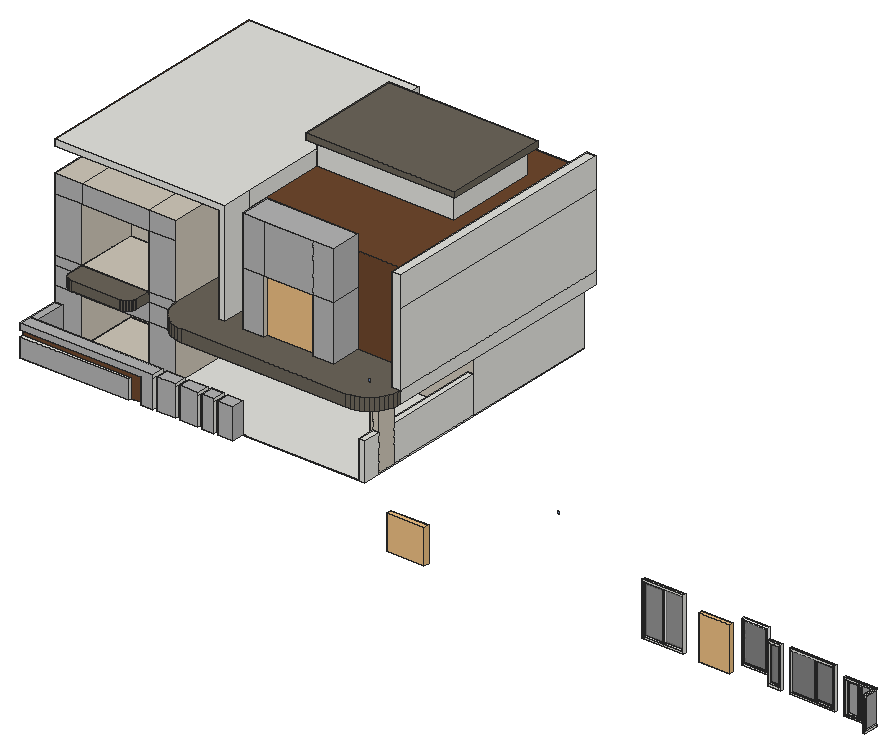
# SketchUp Ruby script. Lengths in millimetres.
U = 1.mm
M = Sketchup.active_model
def pt(a) = Geom::Point3d.new(a.map { |v| v * U })
def face(e, loops, mat)
  f = e.add_face(loops[0].map { |a| pt(a) })
  loops[1..].each { |l| e.add_face(l.map { |a| pt(a) }).erase! }
  f.material = f.back_material = mat if mat
  f
end
# faces: each face lists its corners as indices into pts; further lists are holes
def faces(e, pts, list, mat = nil) = list.each { |f| face(e, (f[0].is_a?(Array) ? f : [f]).map { |l| l.map { |i| pts[i] } }, mat) }
# xy, xz, yz: faces in a plane at the given z, y or x. An outline is a flat list of corners, or four numbers for a rectangle; further outlines are holes
def ring(l) = l.size == 4 ? [[l[0], l[1]], [l[2], l[1]], [l[2], l[3]], [l[0], l[3]]] : l.each_slice(2).to_a
def flat(e, list, mat, &to3) = list.each { |f| face(e, (f[0].is_a?(Array) ? f : [f]).map { |l| ring(l).map { |u, v| to3.(u, v) } }, mat) }
def xy(e, z, list, mat = nil) = flat(e, list, mat) { |x, y| [x, y, z] }
def xz(e, y, list, mat = nil) = flat(e, list, mat) { |x, z| [x, y, z] }
def yz(e, x, list, mat = nil) = flat(e, list, mat) { |y, z| [x, y, z] }
def lines(e, pts, list) = list.each { |a, b| e.add_line(pt(pts[a]), pt(pts[b])) }
# prism: a flat outline (further loops are holes) pulled along v
def prism(e, loops, v, mat = nil)
  f = face(e, loops, mat); d = Geom::Vector3d.new(v.map { |x| x * U })
  f.pushpull(f.normal.samedirection?(d) ? d.length : -d.length)
end
def box(e, o, s, mat = nil) = prism(e, [[o, [o[0] + s[0], o[1], o[2]], [o[0] + s[0], o[1] + s[1], o[2]], [o[0], o[1] + s[1], o[2]]]], [0, 0, s[2]], mat)
def at(x, y, z, deg = 0) = Geom::Transformation.translation(pt([x, y, z])) * Geom::Transformation.rotation(ORIGIN, Z_AXIS, deg.degrees)
def axes(o, x, y, z) = Geom::Transformation.new([*x, 0, *y, 0, *z, 0, *pt(o).to_a, 1])
def part(name) = M.definitions.add(name)
# library, detail: a bought-in or finely detailed component or shape, given as its bounding box
def library(name, o, s) = part(name).tap { |d| box(d.entities, o, s) }
def detail(e, o, s) = box(e.add_group.entities, o, s)
def put(e, d, t, mat = nil) = e.add_instance(d, t).tap { |i| i.material = mat if mat }
def group(e, t, mat = nil) = e.add_group.tap { |g| g.transformation = t; g.material = mat if mat }.entities
root = M.entities
M.materials.add("[0134_DimGray]").color = [107, 101, 90]
M.materials.add("[Beadboard]").color = [109, 71, 45]
M.materials.add("[Carrera Marble]").color = [180, 180, 180]
M.materials.add("[Cinder Block]").color = [206, 198, 184]
M.materials.add("[Color M00]").color = [255, 255, 255]
M.materials.add("[Translucent Glass Gray]1").color = [128, 128, 128]
M.materials["[Translucent Glass Gray]1"].alpha = 0.9
M.materials.add("[Translucent Resin Crush Gray]").color = [165, 165, 165]
M.materials["[Translucent Resin Crush Gray]"].alpha = 1
M.materials.add("[Translucent_Glass_Blue]").color = [100, 149, 237]
M.materials["[Translucent_Glass_Blue]"].alpha = 0.5
c1 = part("Casement window")
xy(c1.entities,0,[[0,0,0,1540,740,1540,740,1440,100,1440,100,0]])
xy(c1.entities,45,[[30,80,100,80,100,1440,660,1440,660,1510,30,1510,30,790,80,790,80,745,30,745]])
xy(c1.entities,70,[[25,815,30,815,30,1510,635,1510,635,1515,25,1515]])
xy(c1.entities,80,[[0,80,10,745],[0,790,10,1540]])
xy(c1.entities,105,[[10,815,15,815,15,1525,635,1525,635,1540,10,1540]])
xy(c1.entities,130,[[25,165,30,660]])
xy(c1.entities,140,[[10,140,15,685]])
xy(c1.entities,1550,[[25,165,30,660]])
xy(c1.entities,1575,[[10,140,15,685]])
xy(c1.entities,1610,[[10,815,10,1540,635,1540,635,1525,15,1525,15,815],[25,815,25,1515,635,1515,635,1510,30,1510,30,815]])
xy(c1.entities,1635,[[0,80,10,745],[30,80,30,745,80,745,80,790,30,790,30,1510,660,1510,660,1440,100,1440,100,80],[0,790,10,1540]])
xy(c1.entities,1715,[[0,0,100,0,100,1440,740,1440,740,1540,0,1540]])
xz(c1.entities,0,[[0,0,100,1715]])
xz(c1.entities,80,[[30,45,100,1635],[0,80,10,1635]])
xz(c1.entities,140,[[10,140,15,1575]])
xz(c1.entities,165,[[25,130,30,1550]])
xz(c1.entities,660,[[25,130,30,1550]])
xz(c1.entities,685,[[10,140,15,1575]])
xz(c1.entities,745,[[30,45,80,1635],[0,80,10,1635]])
xz(c1.entities,790,[[30,45,80,1635],[0,80,10,1635]])
xz(c1.entities,815,[[25,70,30,1610],[10,105,15,1610]])
xz(c1.entities,1440,[[100,0,740,0,740,1715,100,1715,100,1635,660,1635,660,45,100,45]])
xz(c1.entities,1510,[[30,45,660,45,660,1635,30,1635,30,1610,635,1610,635,70,30,70]])
xz(c1.entities,1515,[[25,70,635,1610]],"[Translucent Resin Crush Gray]")
xz(c1.entities,1525,[[15,105,635,1610]],"[Translucent Resin Crush Gray]")
xz(c1.entities,1540,[[0,0,0,80,660,80,660,1635,0,1635,0,1715,740,1715,740,0],[10,80,10,105,635,105,635,1610,10,1610,10,1635,660,1635,660,80]])
yz(c1.entities,0,[[0,0,0,1715,1540,1715,1540,1635,80,1635,80,80,1540,80,1540,0],[745,80,790,1635]])
yz(c1.entities,10,[[[80,80,745,1635],[105,105,720,1610]],[790,80,790,1635,1540,1635,1540,1610,815,1610,815,105,1540,105,1540,80],[[105,105,720,1610],[140,140,685,1575]]])
yz(c1.entities,15,[[815,105,1525,1610],[140,140,685,1575]],"[Translucent Resin Crush Gray]")
yz(c1.entities,25,[[815,70,1515,1610],[165,130,660,1550]],"[Translucent Resin Crush Gray]")
yz(c1.entities,30,[[[80,45,745,1635],[105,70,720,1610]],[790,45,1510,45,1510,70,815,70,815,1610,1510,1610,1510,1635,790,1635],[[105,70,720,1610],[165,130,660,1550]]])
yz(c1.entities,80,[[745,45,790,1635]])
yz(c1.entities,100,[[0,0,1440,0,1440,45,80,45,80,1635,1440,1635,1440,1715,0,1715]])
yz(c1.entities,635,[[1510,70,1515,1610],[1525,105,1540,1610]])
yz(c1.entities,660,[[1440,45,1510,1635]])
yz(c1.entities,740,[[1440,0,1540,1715]])
c2 = library("Group\#97",[0,0,0],[170,1568,2200])
c3 = part("Glass Window Glass Door white frame ประตู หน้าต่าง กรอบขาว")
put(c3.entities,c1,at(10682.2,-611.8,600,-90))
put(c3.entities,c2,at(2888.8,110,0,-90))
g1 = group(c3.entities,at(6847.1,-591.8,600,-90))
xy(g1,0,[[0,0,120,670]])
xy(g1,80,[[0,80,20,590],[50,80,120,590]])
xy(g1,105,[[20,105,25,565],[45,105,50,565]])
xy(g1,170,[[25,170,30,500],[40,170,45,500]])
xy(g1,1860,[[25,170,30,500],[40,170,45,500]])
xy(g1,1925,[[20,105,25,565],[45,105,50,565]])
xy(g1,1950,[[0,80,20,590],[50,80,120,590]])
xy(g1,2030,[[0,0,120,670]])
xz(g1,0,[[0,0,120,2030]])
xz(g1,80,[[0,80,20,1950],[50,80,120,1950]])
xz(g1,105,[[20,105,25,1925],[45,105,50,1925]])
xz(g1,170,[[25,170,30,1860],[40,170,45,1860]])
xz(g1,500,[[25,170,30,1860],[40,170,45,1860]])
xz(g1,565,[[20,105,25,1925],[45,105,50,1925]])
xz(g1,590,[[0,80,20,1950],[50,80,120,1950]])
xz(g1,670,[[0,0,120,2030]])
yz(g1,0,[[[0,0,670,2030],[80,80,590,1950]]])
yz(g1,20,[[[80,80,590,1950],[105,105,565,1925]]])
yz(g1,25,[[[105,105,565,1925],[170,170,500,1860]]])
yz(g1,30,[[170,170,500,1860]],"[Translucent Glass Gray]1")
yz(g1,40,[[170,170,500,1860]],"[Translucent Glass Gray]1")
yz(g1,45,[[[105,105,565,1925],[170,170,500,1860]]])
yz(g1,50,[[[80,80,590,1950],[105,105,565,1925]]])
yz(g1,120,[[[0,0,670,2030],[80,80,590,1950]]])
g2 = group(c3.entities,at(7949.1,-711.8,600))
xy(g2,0,[[0,0,2275,120]])
xy(g2,80,[[80,0,2195,0,2195,57,1280,57,1280,20,1235,20,1235,57,80,57],[80,83,1235,120],[1280,83,2195,120]])
xy(g2,105,[[105,57,1210,65],[105,75,1210,83]])
xy(g2,170,[[1370,57,2105,65],[1370,75,2105,83]])
xy(g2,1890,[[1370,57,2105,65],[1370,75,2105,83]])
xy(g2,1955,[[105,57,1210,65],[105,75,1210,83]])
xy(g2,1980,[[80,0,80,57,1235,57,1235,20,1280,20,1280,57,2195,57,2195,0],[80,83,1235,120],[1280,83,2195,120]])
xy(g2,2060,[[0,0,2275,120]])
xz(g2,0,[[[0,0,2275,2060],[80,80,2195,1980]]])
xz(g2,20,[[1235,80,1280,1980]])
xz(g2,57,[[[80,80,1235,1980],[105,105,1210,1955]],[[1280,80,2195,1980],[1305,105,2170,1955]],[[1305,105,2170,1955],[1370,170,2105,1890]]])
xz(g2,65,[[105,105,1210,1955],[1370,170,2105,1890]],"[Translucent Glass Gray]1")
xz(g2,75,[[105,105,1210,1955],[1370,170,2105,1890]],"[Translucent Glass Gray]1")
xz(g2,83,[[[80,80,1235,1980],[105,105,1210,1955]],[[1280,80,2195,1980],[1305,105,2170,1955]],[[1305,105,2170,1955],[1370,170,2105,1890]]])
xz(g2,120,[[[0,0,2275,2060],[80,80,2195,1980]],[1235,80,1280,1980]])
yz(g2,0,[[0,0,120,2060]])
yz(g2,80,[[0,80,57,1980],[83,80,120,1980]])
yz(g2,105,[[57,105,65,1955],[75,105,83,1955]])
yz(g2,1210,[[57,105,65,1955],[75,105,83,1955]])
yz(g2,1235,[[20,80,57,1980],[83,80,120,1980]])
yz(g2,1280,[[20,80,57,1980],[83,80,120,1980]])
yz(g2,1370,[[57,170,65,1890],[75,170,83,1890]])
yz(g2,2105,[[57,170,65,1890],[75,170,83,1890]])
yz(g2,2195,[[0,80,57,1980],[83,80,120,1980]])
yz(g2,2275,[[0,0,120,2060]])
g3 = group(c3.entities,at(0,0,0))
xy(g3,0,[[0,0,80,140],[2010,0,2050,140],[80,20,2010,120]])
xy(g3,85,[[80,20,2010,120]],"[Color M00]")
xy(g3,2565,[[80,0,2010,140]])
xy(g3,2650,[[0,0,2050,140]])
xz(g3,0,[[0,0,80,0,80,2565,2010,2565,2010,0,2050,0,2050,2650,0,2650]])
xz(g3,20,[[80,0,2010,85]])
xz(g3,120,[[80,0,2010,85]])
xz(g3,140,[[0,0,0,2650,2050,2650,2050,0,2010,0,2010,2565,80,2565,80,0]])
yz(g3,0,[[0,0,140,2650]])
yz(g3,80,[[0,0,20,0,20,85,120,85,120,0,140,0,140,2565,0,2565],[20,0,120,85]])
yz(g3,2010,[[0,0,0,2565,140,2565,140,0,120,0,120,85,20,85,20,0],[20,0,120,85]])
yz(g3,2050,[[0,0,140,2650]])
g4 = group(g3,at(80,20,85))
g5 = group(g4,at(940,50,0))
xy(g5,0,[[0,0,990,50]],"[Color M00]")
xy(g5,60,[[60,0,940,30],[60,30,940,50]],"[Color M00]")
xy(g5,2420,[[60,0,940,30],[60,30,940,50]],"[Color M00]")
xy(g5,2480,[[0,0,990,50]],"[Color M00]")
xz(g5,0,[[[0,0,990,2480],[60,60,940,2420]]],"[Color M00]")
xz(g5,30,[[60,60,940,2420]],"[Translucent Glass Gray]1")
xz(g5,50,[[[0,0,990,2480],[60,60,940,2420]]],"[Color M00]")
yz(g5,0,[[0,0,50,2480]],"[Color M00]")
yz(g5,60,[[0,60,30,2420],[30,60,50,2420]],"[Color M00]")
yz(g5,940,[[0,60,30,2420],[30,60,50,2420]],"[Color M00]")
yz(g5,990,[[0,0,50,2480]],"[Color M00]")
g6 = group(g4,at(0,0,0))
xy(g6,0,[[0,0,990,50]],"[Color M00]")
xy(g6,60,[[60,0,940,30],[60,30,940,50]],"[Color M00]")
xy(g6,2420,[[60,0,940,30],[60,30,940,50]],"[Color M00]")
xy(g6,2480,[[0,0,990,50]],"[Color M00]")
xz(g6,0,[[[0,0,990,2480],[60,60,940,2420]]],"[Color M00]")
xz(g6,30,[[60,60,940,2420]],"[Translucent Glass Gray]1")
xz(g6,50,[[[0,0,990,2480],[60,60,940,2420]]],"[Color M00]")
yz(g6,0,[[0,0,50,2480]],"[Color M00]")
yz(g6,60,[[0,60,30,2420],[30,60,50,2420]],"[Color M00]")
yz(g6,940,[[0,60,30,2420],[30,60,50,2420]],"[Color M00]")
yz(g6,990,[[0,0,50,2480]],"[Color M00]")
g7 = group(c3.entities,at(5008,0,560))
xy(g7,0,[[0,0,1280,120]],"[Color M00]")
xy(g7,80,[[80,0,1200,60],[80,80,1200,120]],"[Color M00]")
xy(g7,105,[[105,60,1175,65],[105,65,1175,75],[105,75,1175,80]],"[Color M00]")
xy(g7,1985,[[105,60,1175,65],[105,65,1175,75],[105,75,1175,80]],"[Color M00]")
xy(g7,2010,[[80,0,1200,60],[80,80,1200,120]],"[Color M00]")
xy(g7,2090,[[0,0,1280,120]],"[Color M00]")
xz(g7,0,[[[0,0,1280,2090],[80,80,1200,2010]]],"[Color M00]")
xz(g7,60,[[[80,80,1200,2010],[105,105,1175,1985]]],"[Color M00]")
xz(g7,65,[[105,105,1175,1985]],"[Translucent Glass Gray]1")
xz(g7,75,[[105,105,1175,1985]],"[Translucent Glass Gray]1")
xz(g7,80,[[[80,80,1200,2010],[105,105,1175,1985]]],"[Color M00]")
xz(g7,120,[[[0,0,1280,2090],[80,80,1200,2010]]],"[Color M00]")
yz(g7,0,[[0,0,120,2090]],"[Color M00]")
yz(g7,80,[[0,80,60,2010],[80,80,120,2010]],"[Color M00]")
yz(g7,105,[[60,105,65,1985],[65,105,75,1985],[75,105,80,1985]],"[Color M00]")
yz(g7,1175,[[60,105,65,1985],[65,105,75,1985],[75,105,80,1985]],"[Color M00]")
yz(g7,1200,[[0,80,60,2010],[80,80,120,2010]],"[Color M00]")
yz(g7,1280,[[0,0,120,2090]],"[Color M00]")
c4 = part("Picture Frame Glass")
box(c4.entities,[0,0,0],[101.6,3.2,152.4],"[Translucent_Glass_Blue]")
c5 = library("Group\#16",[0,0,0],[3156.4,444.1,2863.6])
xy(root,-13.9,[[0,1351.8,6092.9,2875.8]])
xy(root,-10.7,[[0,742.2,0,1351.8,10668,1351.8,10668,742.2,9906,742.2,9906,894.6,9702.8,894.6,9702.8,742.2,9093.2,742.2,9093.2,894.6,8890,894.6,8890,742.2,7975.6,742.2,7975.6,894.6,7772.4,894.6,7772.4,742.2,6858,742.2,6858,894.6,6654.8,894.6,6654.8,742.2,6045.2,742.2,6045.2,894.6,5435.6,894.6,5435.6,742.2],[[0,1351.8,16764,15067.8],[1371.6,2875.8,4721.3,5923.8]]])
xy(root,14.7,[[0,1351.8,408.5,2875.8],[408.5,1351.8,6092.9,2875.8],[6092.9,1351.8,16459.2,1351.8,16459.2,2266.2,16306.8,2266.2,16306.8,3180.6,16459.2,3180.6,16459.2,8209.8,11579.3,8209.8,11579.3,11257.8,10360.1,11257.8,10360.1,8209.8,9140.9,8209.8,9140.9,5923.8,6092.9,5923.8],[16306.8,2266.2,16764,3180.6],[0,2875.8,0,15067.8,16764,15067.8,16764,8209.8,11579.3,8209.8,11579.3,11257.8,10360.1,11257.8,10360.1,8209.8,6092.9,8209.8,6092.9,2875.8,4721.3,2875.8,4721.3,5923.8,1371.6,5923.8,1371.6,2875.8],
  [16459.2,3180.6,16764,8209.8],[6092.9,5923.8,9140.9,8057.4],[6092.9,8057.4,9140.9,8209.8]])
xy(root,14.7,[[1371.6,2875.8,4721.3,5923.8]],"[Cinder Block]")
xy(root,929.1,[[0,742.2,5435.6,894.6]])
xy(root,1233.9,[[0,742.2,6045.2,894.6]])
xy(root,1386.3,[[6654.8,894.6,6858,1351.8],[7772.4,894.6,7975.6,1351.8],[8890,894.6,9093.2,1351.8],[9702.8,894.6,9906,1351.8]],"[Beadboard]")
xy(root,1538.7,[[0,742.2,6654.8,1351.8],[6858,742.2,7772.4,1351.8],[7975.6,742.2,8890,1351.8],[9093.2,742.2,9702.8,1351.8],[9906,742.2,10668,1351.8],
  [0,1351.8,408.5,2875.8]],"[Carrera Marble]")
xy(root,1843.5,[[16459.2,1351.8,16764,2266.2],[16459.2,3180.6,16764,8209.8]])
xy(root,1843.5,[[14322.5,8209.8,14932.1,9733.8]],"[Cinder Block]")
xy(root,2300.7,[[1371.6,2875.8,4721.3,5923.8]])
xy(root,2453.1,[[10360.1,8209.8,11579.3,11257.8],[14322.5,8209.8,14932.1,9733.8]],"[Cinder Block]")
xy(root,3062.7,[[7616.9,1351.8,7418,1364.8,7222.5,1403.7,7033.7,1467.8,6854.9,1555.9,6689.2,1666.7,6539.3,1798.1,6407.9,1948,6297.1,2113.8,6209,2292.5,6144.9,2481.3,6106,2676.8,6092.9,2875.8,6092.9,5923.8,9140.9,5923.8,9140.9,8209.8,17373.6,8209.8,17373.6,3180.6,16764,3180.6,16764,2266.2,17244.6,2266.2,17169.4,2113.8,17058.7,1948,16927.2,1798.1,16777.4,1666.7,16611.6,1555.9,16432.8,1467.8,16244,1403.7,16048.5,1364.8,15849.6,1351.8],[16764,2266.2,17244.6,2266.2,17257.6,2292.5,17321.7,2481.3,17360.6,2676.8,17373.6,2875.8,17373.6,3180.6,16764,3180.6],[6092.9,5923.8,9140.9,8057.4],[6092.9,8057.4,9140.9,8209.8],[16764,8209.8,17373.6,15067.8]])
xy(root,3123,[[16306.8,2266.2,16764,3180.6]])
xy(root,3215.1,[[1828.8,1656.6,1769.1,1660.5,1710.5,1672.1,1653.8,1691.4,1600.2,1717.8,1550.5,1751,1505.5,1790.5,1466.1,1835.4,1432.9,1885.2,1406.4,1938.8,1387.2,1995.4,1375.5,2054.1,1371.6,2113.8,1371.6,2875.8,4721.3,2875.8,4721.3,2113.8,4717.4,2054.1,4705.8,1995.4,4686.5,1938.8,4660.1,1885.2,4626.9,1835.4,4587.4,1790.5,4542.5,1751,4492.7,1717.8,4439.1,1691.4,4382.5,1672.1,4323.8,1660.5,4264.1,1656.6]])
xy(root,3559.6,[[1371.6,2875.8,4721.3,5923.8]])
xy(root,3672.3,[[0,2875.8,0,15067.8,17373.6,15067.8,17373.6,2875.8,16916.4,2875.8,16916.4,4399.8,14017.7,4399.8,14017.7,2875.8,12950.9,2875.8,12950.9,4399.8,10512.5,4399.8,10512.5,2875.8,9445.7,2875.8,9445.7,4399.8,8531.3,4399.8,8531.3,2875.8,8226.5,2875.8,8226.5,5923.8,6092.9,5923.8,6092.9,2875.8,4721.3,2875.8,4721.3,5923.8,1371.6,5923.8,1371.6,2875.8]])
xy(root,3672.3,[[7616.9,1351.8,15849.6,1351.8,16048.5,1364.8,16244,1403.7,16432.8,1467.8,16611.6,1555.9,16777.4,1666.7,16927.2,1798.1,17058.7,1948,17169.4,2113.8,17257.6,2292.5,17321.7,2481.3,17360.6,2676.8,17373.6,2875.8,16916.4,2875.8,16916.4,4399.8,14017.7,4399.8,14017.7,2875.8,12950.9,2875.8,12950.9,4399.8,10512.5,4399.8,10512.5,2875.8,9445.7,2875.8,9445.7,4399.8,8531.3,4399.8,8531.3,2875.8,8226.5,2875.8,8226.5,5923.8,6092.9,5923.8,6092.9,2875.8,6106,2676.8,6144.9,2481.3,6209,2292.5,6297.1,2113.8,6407.9,1948,6539.3,1798.1,6689.2,1666.7,6854.9,1555.9,7033.7,1467.8,7222.5,1403.7,7418,1364.8],[1828.8,1656.6,4264.1,1656.6,4323.8,1660.5,4382.5,1672.1,4439.1,1691.4,4492.7,1717.8,4542.5,1751,4587.4,1790.5,4626.9,1835.4,4660.1,1885.2,4686.5,1938.8,4705.8,1995.4,4717.4,2054.1,4721.3,2113.8,4721.3,2875.8,1371.6,2875.8,1371.6,2113.8,1375.5,2054.1,1387.2,1995.4,1406.4,1938.8,1432.9,1885.2,1466.1,1835.4,1505.5,1790.5,1550.5,1751,1600.2,1717.8,1653.8,1691.4,1710.5,1672.1,1769.1,1660.5]],"[0134_DimGray]")
xy(root,3672.3,[[1371.6,2875.8,4721.3,5923.8]],"[Cinder Block]")
xy(root,6415.5,[[1371.6,2875.8,4721.3,5923.8],[10512.5,2875.8,12950.9,4399.8]],"[Cinder Block]")
xy(root,7329.9,[[0,2875.8,1371.6,5923.8],[1371.6,2875.8,4721.3,5923.8],[4721.3,2875.8,6092.9,5923.8]],"[Cinder Block]")
xy(root,8091.9,[[8531.3,8667,15392.4,13239]])
xy(root,8091.9,[[8531.3,4399.8,16916.4,4399.8,16916.4,15067.8,8531.3,15067.8,8531.3,13239,15392.4,13239,15392.4,8667,8531.3,8667]],"[Beadboard]")
xy(root,8549.1,[[0,2875.8,8226.5,5923.8]])
xy(root,8853.9,[[0,2875.8,8531.3,15067.8],[16916.4,2875.8,17373.6,15067.8]])
xy(root,8853.9,[[9445.7,2875.8,14017.7,4399.8]],"[Carrera Marble]")
xy(root,9311.1,[[8531.3,8667,15392.4,13239]])
xy(root,9311.1,[[8226.5,8362.2,15697.2,8667],[8226.5,8667,8531.3,13543.8],[15392.4,8667,15697.2,13543.8],[8531.3,13239,15392.4,13543.8]],"[0134_DimGray]")
xy(root,9615.9,[[8226.5,8362.2,15697.2,13543.8]],"[0134_DimGray]")
xz(root,742.2,[[0,-10.7,5435.6,929.1],[6045.2,-10.7,6654.8,-10.7,6654.8,1538.7,0,1538.7,0,1233.9,6045.2,1233.9],[6858,-10.7,7772.4,1538.7],[7975.6,-10.7,8890,1538.7],[9093.2,-10.7,9702.8,1538.7],
  [9906,-10.7,10668,1538.7]],"[Carrera Marble]")
xz(root,894.6,[[5435.6,-10.7,6045.2,-10.7,6045.2,1233.9,0,1233.9,0,929.1,5435.6,929.1],[6654.8,-10.7,6858,1386.3],[7772.4,-10.7,7975.6,1386.3],[8890,-10.7,9093.2,1386.3],[9702.8,-10.7,9906,1386.3]],"[Beadboard]")
xz(root,1351.8,[[0,-13.9,6092.9,-10.7],[0,-10.7,6092.9,14.7],[6092.9,-10.7,10668,14.7],[10668,-10.7,16764,-10.7,16764,1843.5,16459.2,1843.5,16459.2,14.7,10668,14.7],[0,14.7,408.5,1538.7],
  [6092.9,14.7,6092.9,1538.7,6654.8,1538.7,6654.8,1386.3,6858,1386.3,6858,1538.7,7772.4,1538.7,7772.4,1386.3,7975.6,1386.3,7975.6,1538.7,8890,1538.7,8890,1386.3,9093.2,1386.3,9093.2,1538.7,9702.8,1538.7,9702.8,1386.3,9906,1386.3,9906,1538.7,10668,1538.7,10668,14.7]])
xz(root,1351.8,[[7616.9,3062.7,15849.6,3672.3]],"[0134_DimGray]")
xz(root,1351.8,[[408.5,14.7,6092.9,1538.7]],"[Carrera Marble]")
xz(root,1656.6,[[1828.8,3215.1,4264.1,3672.3]],"[0134_DimGray]")
xz(root,2266.2,[[16459.2,14.7,16764,1843.5]])
xz(root,2266.2,[[16306.8,14.7,16459.2,3123],[16459.2,1843.5,16764,3123]],"[Cinder Block]")
xz(root,2875.8,[[0,-13.9,0,14.7,1371.6,14.7,1371.6,-10.7,4721.3,-10.7,4721.3,14.7,6092.9,14.7,6092.9,-13.9],[1371.6,-10.7,4721.3,14.7],[0,14.7,408.5,1538.7],[1371.6,3215.1,4721.3,3559.6],[1371.6,3559.6,4721.3,3672.3],
  [8226.5,3672.3,8531.3,3672.3,8531.3,8853.9,0,8853.9,0,8549.1,8226.5,8549.1],[16916.4,3672.3,17373.6,8853.9]])
xz(root,2875.8,[[408.5,14.7,1371.6,14.7,1371.6,2300.7,0,2300.7,0,1538.7,408.5,1538.7],[4721.3,14.7,6092.9,2300.7],[0,2300.7,1371.6,3215.1],[1371.6,2300.7,4721.3,3215.1],[4721.3,2300.7,6092.9,3215.1],
  [0,3215.1,1371.6,3672.3],[4721.3,3215.1,6092.9,3672.3],[0,3672.3,1371.6,6415.5],[4721.3,3672.3,6092.9,6415.5],[9445.7,3672.3,10512.5,6415.5],
  [12950.9,3672.3,14017.7,6415.5],[0,6415.5,1371.6,7329.9],[1371.6,6415.5,4721.3,7329.9],[4721.3,6415.5,6092.9,7329.9],[9445.7,6415.5,10512.5,8853.9],
  [10512.5,6415.5,12950.9,8853.9],[12950.9,6415.5,14017.7,8853.9]],"[Carrera Marble]")
xz(root,3180.6,[[16459.2,14.7,16764,1843.5]])
xz(root,3180.6,[[16306.8,14.7,16459.2,3123],[16459.2,1843.5,16764,3123]],"[Cinder Block]")
xz(root,4399.8,[[9445.7,8091.9,14017.7,8853.9]])
xz(root,4399.8,[[8531.3,3672.3,9445.7,8091.9],[14017.7,3672.3,16916.4,8091.9]],"[Beadboard]")
xz(root,4399.8,[[10512.5,3672.3,12950.9,6415.5]],"[Cinder Block]")
xz(root,5923.8,[[1371.6,-10.7,4721.3,14.7],[1371.6,3559.6,4721.3,3672.3]])
xz(root,5923.8,[[6092.9,14.7,9140.9,3062.7],[6092.9,3672.3,8226.5,3672.3,8226.5,8549.1,0,8549.1,0,7329.9,6092.9,7329.9]],"[Beadboard]")
xz(root,5923.8,[[1371.6,14.7,4721.3,2300.7],[1371.6,3672.3,4721.3,6415.5]],"[Cinder Block]")
xz(root,8209.8,[[6092.9,14.7,9140.9,3062.7],[16459.2,14.7,16764,1843.5]])
xz(root,8209.8,[[[9140.9,14.7,10360.1,14.7,10360.1,2453.1,11579.3,2453.1,11579.3,14.7,16459.2,14.7,16459.2,1843.5,16764,1843.5,16764,3062.7,9140.9,3062.7],[14322.5,1843.5,14932.1,2453.1]]],"[Cinder Block]")
xz(root,8362.2,[[8226.5,9311.1,15697.2,9615.9]],"[0134_DimGray]")
xz(root,8667,[[8531.3,8091.9,15392.4,9311.1]])
xz(root,9733.8,[[14322.5,1843.5,14932.1,2453.1]],"[Cinder Block]")
xz(root,11257.8,[[10360.1,14.7,11579.3,2453.1]],"[Cinder Block]")
xz(root,13239,[[8531.3,8091.9,15392.4,9311.1]])
xz(root,13543.8,[[8226.5,9311.1,15697.2,9615.9]],"[0134_DimGray]")
xz(root,15067.8,[[0,-10.7,16764,14.7],[0,14.7,16764,3062.7],[0,3062.7,17373.6,3672.3],[0,3672.3,17373.6,7329.9],[0,7329.9,0,8853.9,8531.3,8853.9,8531.3,8091.9,16916.4,8091.9,16916.4,8853.9,17373.6,8853.9,17373.6,7329.9]])
yz(root,0,[[1351.8,-13.9,2875.8,-10.7],[742.2,-10.7,742.2,929.1,894.6,929.1,894.6,1233.9,742.2,1233.9,742.2,1538.7,1351.8,1538.7,1351.8,-10.7],[1351.8,-10.7,2875.8,14.7],[2875.8,-10.7,15067.8,14.7],[1351.8,14.7,2875.8,1538.7]])
yz(root,0,[[5923.8,7329.9,5923.8,8549.1,2875.8,8549.1,2875.8,8853.9,15067.8,8853.9,15067.8,7329.9]],"[Beadboard]")
yz(root,0,[[2875.8,14.7,15067.8,3062.7],[2875.8,3062.7,15067.8,3672.3],[2875.8,3672.3,15067.8,7329.9]],"[Carrera Marble]")
yz(root,408.5,[[1351.8,14.7,2875.8,1538.7]],"[Carrera Marble]")
yz(root,1371.6,[[2875.8,-10.7,5923.8,14.7],[2875.8,3559.6,5923.8,3672.3]])
yz(root,1371.6,[[2113.8,3215.1,2875.8,3672.3]],"[0134_DimGray]")
yz(root,1371.6,[[2875.8,14.7,5923.8,2300.7],[2875.8,3672.3,5923.8,6415.5]],"[Cinder Block]")
yz(root,4721.3,[[2875.8,-10.7,5923.8,14.7],[2875.8,3559.6,5923.8,3672.3]])
yz(root,4721.3,[[2113.8,3215.1,2875.8,3672.3]],"[0134_DimGray]")
yz(root,4721.3,[[2875.8,14.7,5923.8,2300.7],[2875.8,3672.3,5923.8,6415.5]],"[Cinder Block]")
yz(root,5435.6,[[742.2,-10.7,894.6,929.1]])
yz(root,6045.2,[[742.2,-10.7,894.6,1233.9]])
yz(root,6092.9,[[1351.8,-13.9,2875.8,14.7],[5923.8,14.7,8057.4,3062.7],[8057.4,14.7,8209.8,3062.7]])
yz(root,6092.9,[[2875.8,14.7,5923.8,3062.7],[2875.8,3672.3,5923.8,7329.9]],"[Cinder Block]")
yz(root,6654.8,[[742.2,-10.7,894.6,1386.3],[742.2,1386.3,1351.8,1538.7]])
yz(root,6858,[[742.2,-10.7,894.6,1386.3],[742.2,1386.3,1351.8,1538.7]])
yz(root,7772.4,[[742.2,-10.7,894.6,1386.3],[742.2,1386.3,1351.8,1538.7]])
yz(root,7975.6,[[742.2,-10.7,894.6,1386.3],[742.2,1386.3,1351.8,1538.7]])
yz(root,8226.5,[[2875.8,3672.3,5923.8,8549.1]])
yz(root,8226.5,[[8362.2,9311.1,13543.8,9615.9]],"[0134_DimGray]")
yz(root,8531.3,[[2875.8,3672.3,4399.8,8853.9],[4399.8,8091.9,8667,8853.9],[8667,8091.9,13239,8853.9],[13239,8091.9,15067.8,8853.9],[8667,8853.9,13239,9311.1]])
yz(root,8890,[[742.2,-10.7,894.6,1386.3],[742.2,1386.3,1351.8,1538.7]])
yz(root,9093.2,[[742.2,-10.7,894.6,1386.3],[742.2,1386.3,1351.8,1538.7]])
yz(root,9140.9,[[5923.8,14.7,8209.8,3062.7]],"[Beadboard]")
yz(root,9445.7,[[2875.8,3672.3,4399.8,6415.5],[2875.8,6415.5,4399.8,8853.9]],"[Carrera Marble]")
yz(root,9702.8,[[742.2,-10.7,894.6,1386.3],[742.2,1386.3,1351.8,1538.7]])
yz(root,9906,[[742.2,-10.7,894.6,1386.3],[742.2,1386.3,1351.8,1538.7]])
yz(root,10360.1,[[8209.8,14.7,11257.8,2453.1]],"[Cinder Block]")
yz(root,10512.5,[[2875.8,3672.3,4399.8,6415.5]],"[Cinder Block]")
yz(root,10668,[[742.2,-10.7,1351.8,1538.7]],"[Carrera Marble]")
yz(root,11579.3,[[8209.8,14.7,11257.8,2453.1]],"[Cinder Block]")
yz(root,12950.9,[[2875.8,3672.3,4399.8,6415.5]],"[Cinder Block]")
yz(root,14017.7,[[2875.8,3672.3,4399.8,6415.5],[2875.8,6415.5,4399.8,8853.9]],"[Carrera Marble]")
yz(root,14322.5,[[8209.8,1843.5,9733.8,2453.1]],"[Cinder Block]")
yz(root,14932.1,[[8209.8,1843.5,9733.8,2453.1]],"[Cinder Block]")
yz(root,15392.4,[[8667,8091.9,13239,9311.1]])
yz(root,15697.2,[[8362.2,9311.1,13543.8,9615.9]],"[0134_DimGray]")
yz(root,16306.8,[[2266.2,14.7,3180.6,3123]],"[Cinder Block]")
yz(root,16459.2,[[1351.8,14.7,2266.2,1843.5],[3180.6,14.7,8209.8,1843.5]])
yz(root,16764,[[1351.8,-10.7,15067.8,-10.7,15067.8,14.7,2266.2,14.7,2266.2,1843.5,1351.8,1843.5],[3180.6,14.7,8209.8,1843.5],[8209.8,14.7,15067.8,3062.7],[2266.2,3062.7,3180.6,3123]])
yz(root,16764,[[2266.2,14.7,3180.6,3062.7]],"[Cinder Block]")
yz(root,16916.4,[[2875.8,3672.3,4399.8,8853.9],[4399.8,8091.9,15067.8,8853.9]])
yz(root,17373.6,[[2875.8,3062.7,15067.8,3672.3],[2875.8,3672.3,15067.8,7329.9],[2875.8,7329.9,15067.8,8853.9]])
p = [[7616.9,1351.8,3672.3],[7418,1364.8,3672.3],[7418,1364.8,3062.7],[7616.9,1351.8,3062.7],[16048.5,1364.8,3672.3],[15849.6,1351.8,3672.3],
  [15849.6,1351.8,3062.7],[16048.5,1364.8,3062.7],[7222.5,1403.7,3672.3],[7222.5,1403.7,3062.7],[16244,1403.7,3672.3],[16244,1403.7,3062.7],
  [7033.7,1467.8,3672.3],[7033.7,1467.8,3062.7],[16432.8,1467.8,3672.3],[16432.8,1467.8,3062.7],[6854.9,1555.9,3672.3],[6854.9,1555.9,3062.7],
  [16611.6,1555.9,3672.3],[16611.6,1555.9,3062.7],[6689.2,1666.7,3672.3],[6689.2,1666.7,3062.7],[16777.4,1666.7,3672.3],[16777.4,1666.7,3062.7],
  [6539.3,1798.1,3672.3],[6539.3,1798.1,3062.7],[16927.2,1798.1,3672.3],[16927.2,1798.1,3062.7],[6407.9,1948,3672.3],[6407.9,1948,3062.7],
  [17058.7,1948,3672.3],[17058.7,1948,3062.7],[6297.1,2113.8,3672.3],[6297.1,2113.8,3062.7],[17169.4,2113.8,3672.3],[17169.4,2113.8,3062.7],
  [6209,2292.5,3672.3],[6209,2292.5,3062.7],[17244.6,2266.2,3062.7],[17257.6,2292.5,3062.7],[17257.6,2292.5,3672.3],[6144.9,2481.3,3672.3],
  [6144.9,2481.3,3062.7],[17321.7,2481.3,3062.7],[17321.7,2481.3,3672.3],[6106,2676.8,3672.3],[6106,2676.8,3062.7],[17360.6,2676.8,3062.7],
  [17360.6,2676.8,3672.3],[6092.9,2875.8,3672.3],[6092.9,2875.8,3215.1],[6092.9,2875.8,3062.7],[17373.6,2875.8,3062.7],[17373.6,2875.8,3672.3],
  [1828.8,1656.6,3672.3],[1769.1,1660.5,3672.3],[1769.1,1660.5,3215.1],[1828.8,1656.6,3215.1],[4323.8,1660.5,3672.3],[4264.1,1656.6,3672.3],
  [4264.1,1656.6,3215.1],[4323.8,1660.5,3215.1],[1710.5,1672.1,3672.3],[1710.5,1672.1,3215.1],[4382.5,1672.1,3672.3],[4382.5,1672.1,3215.1],
  [1653.8,1691.4,3672.3],[1653.8,1691.4,3215.1],[4439.1,1691.4,3672.3],[4439.1,1691.4,3215.1],[1600.2,1717.8,3672.3],[1600.2,1717.8,3215.1],
  [4492.7,1717.8,3672.3],[4492.7,1717.8,3215.1],[1550.5,1751,3672.3],[1550.5,1751,3215.1],[4542.5,1751,3672.3],[4542.5,1751,3215.1],
  [1505.5,1790.5,3672.3],[1505.5,1790.5,3215.1],[4587.4,1790.5,3672.3],[4587.4,1790.5,3215.1],[1466.1,1835.4,3672.3],[1466.1,1835.4,3215.1],
  [4626.9,1835.4,3672.3],[4626.9,1835.4,3215.1],[1432.9,1885.2,3672.3],[1432.9,1885.2,3215.1],[4660.1,1885.2,3672.3],[4660.1,1885.2,3215.1],
  [1406.4,1938.8,3672.3],[1406.4,1938.8,3215.1],[4686.5,1938.8,3672.3],[4686.5,1938.8,3215.1],[1387.2,1995.4,3672.3],[1387.2,1995.4,3215.1],
  [4705.8,1995.4,3672.3],[4705.8,1995.4,3215.1],[1375.5,2054.1,3672.3],[1375.5,2054.1,3215.1],[4717.4,2054.1,3672.3],[4717.4,2054.1,3215.1],
  [1371.6,2113.8,3672.3],[1371.6,2113.8,3215.1],[4721.3,2113.8,3672.3],[4721.3,2113.8,3215.1]]
faces(root,p,[[0,1,2,3],[4,5,6,7],[1,8,9,2],[10,4,7,11],[8,12,13,9],[14,10,11,15],[12,16,17,13],[18,14,15,19],
  [16,20,21,17],[22,18,19,23],[20,24,25,21],[26,22,23,27],[24,28,29,25],[30,26,27,31],[28,32,33,29],[34,30,31,35],
  [32,36,37,33],[35,38,39,40,34],[36,41,42,37],[40,39,43,44],[41,45,46,42],[44,43,47,48],[45,49,50,51,46],[48,47,52,53],
  [54,55,56,57],[58,59,60,61],[55,62,63,56],[64,58,61,65],[62,66,67,63],[68,64,65,69],[66,70,71,67],[72,68,69,73],
  [70,74,75,71],[76,72,73,77],[74,78,79,75],[80,76,77,81],[78,82,83,79],[84,80,81,85],[82,86,87,83],[88,84,85,89],
  [86,90,91,87],[92,88,89,93],[90,94,95,91],[96,92,93,97],[94,98,99,95],[100,96,97,101],[98,102,103,99],[104,100,101,105]],"[0134_DimGray]")
put(root,c3,at(30690.6,1351.8,-2107.8))
put(root,c4,at(26470.4,1351.8,1974.8))
put(root,c4,at(16995.9,1351.8,4593.5))
put(root,c5,axes([18051.1,1126,-2541.1],[0.6,0,0],[0,0.6,0],[0,0,0.6]))
put(root,c5,axes([10511.2,3066.2,3672.3],[0.768,0,0],[0,0.768,0],[0,0,0.94385]))
